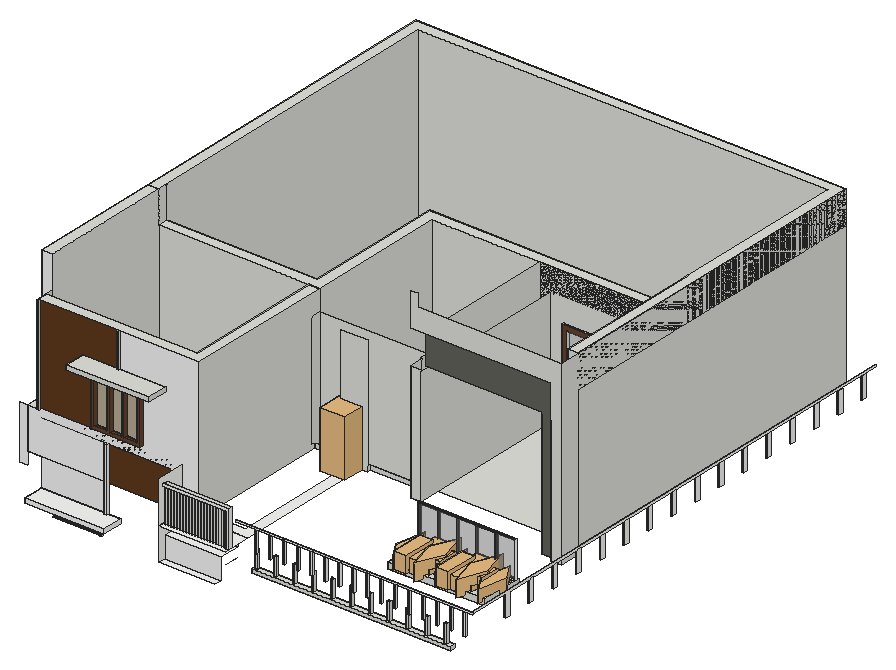
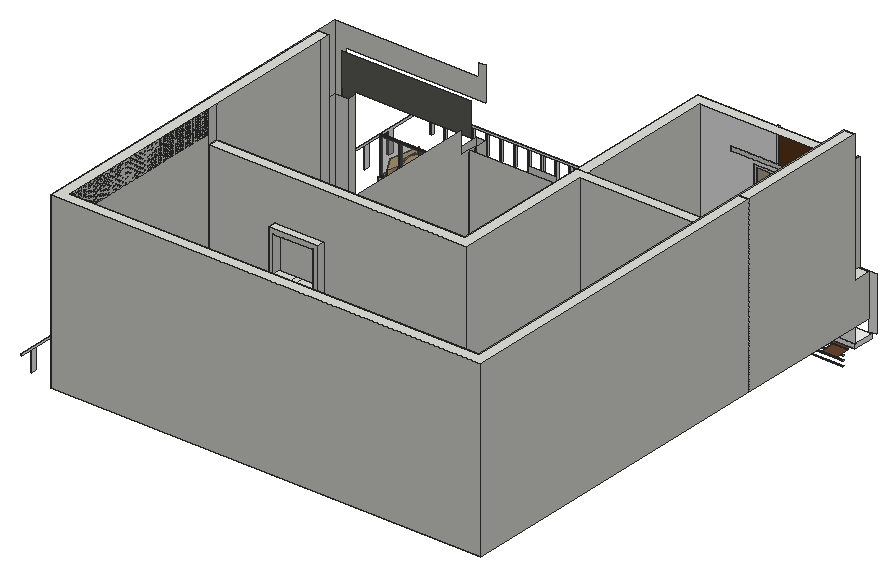
# SketchUp Ruby script. Lengths in inches.
U = 1.inch
M = Sketchup.active_model
def pt(a) = Geom::Point3d.new(a.map { |v| v * U })
def face(e, loops, mat)
  f = e.add_face(loops[0].map { |a| pt(a) })
  loops[1..].each { |l| e.add_face(l.map { |a| pt(a) }).erase! }
  f.material = f.back_material = mat if mat
  f
end
# faces: each face lists its corners as indices into pts; further lists are holes
def faces(e, pts, list, mat = nil) = list.each { |f| face(e, (f[0].is_a?(Array) ? f : [f]).map { |l| l.map { |i| pts[i] } }, mat) }
# xy, xz, yz: faces in a plane at the given z, y or x. An outline is a flat list of corners, or four numbers for a rectangle; further outlines are holes
def ring(l) = l.size == 4 ? [[l[0], l[1]], [l[2], l[1]], [l[2], l[3]], [l[0], l[3]]] : l.each_slice(2).to_a
def flat(e, list, mat, &to3) = list.each { |f| face(e, (f[0].is_a?(Array) ? f : [f]).map { |l| ring(l).map { |u, v| to3.(u, v) } }, mat) }
def xy(e, z, list, mat = nil) = flat(e, list, mat) { |x, y| [x, y, z] }
def xz(e, y, list, mat = nil) = flat(e, list, mat) { |x, z| [x, y, z] }
def yz(e, x, list, mat = nil) = flat(e, list, mat) { |y, z| [x, y, z] }
def lines(e, pts, list) = list.each { |a, b| e.add_line(pt(pts[a]), pt(pts[b])) }
# prism: a flat outline (further loops are holes) pulled along v
def prism(e, loops, v, mat = nil)
  f = face(e, loops, mat); d = Geom::Vector3d.new(v.map { |x| x * U })
  f.pushpull(f.normal.samedirection?(d) ? d.length : -d.length)
end
def box(e, o, s, mat = nil) = prism(e, [[o, [o[0] + s[0], o[1], o[2]], [o[0] + s[0], o[1] + s[1], o[2]], [o[0], o[1] + s[1], o[2]]]], [0, 0, s[2]], mat)
def at(x, y, z, deg = 0) = Geom::Transformation.translation(pt([x, y, z])) * Geom::Transformation.rotation(ORIGIN, Z_AXIS, deg.degrees)
def axes(o, x, y, z) = Geom::Transformation.new([*x, 0, *y, 0, *z, 0, *pt(o).to_a, 1])
def part(name) = M.definitions.add(name)
# library, detail: a bought-in or finely detailed component or shape, given as its bounding box
def library(name, o, s) = part(name).tap { |d| box(d.entities, o, s) }
def detail(e, o, s) = box(e.add_group.entities, o, s)
def put(e, d, t, mat = nil) = e.add_instance(d, t).tap { |i| i.material = mat if mat }
def group(e, t, mat = nil) = e.add_group.tap { |g| g.transformation = t; g.material = mat if mat }.entities
root = M.entities
M.materials.add("ARMANI GRIS").color = [109, 100, 95]
M.materials.add("Brick_21_1K").color = [96, 58, 28]
M.materials.add("CALACATA").color = [248, 248, 247]
M.materials.add("Glass_Basic_01").color = [161, 173, 186]
M.materials["Glass_Basic_01"].alpha = 0.25
M.materials.add("Glass_Mirror_1").color = [185, 173, 151]
M.materials.add("Glass_Safety_01").color = [204, 235, 244]
M.materials["Glass_Safety_01"].alpha = 0.25
M.materials.add("Material__1").color = [95, 70, 46]
M.materials.add("Metal_06_1K").color = [238, 236, 231]
M.materials.add("PIETRA GRAY").color = [98, 99, 92]
M.materials.add("Wood_Veneer_15_1K").color = [103, 69, 45]
M.materials.add("[Color M00]").color = [255, 255, 255]
M.materials.add("[Translucent Glass Gray]").color = [128, 128, 128]
M.materials["[Translucent Glass Gray]"].alpha = 0.29
c1 = library("Group_2",[-1.28,-0.39,0],[21.22,20.51,48.44])
c2 = library("Areca palm plant",[0,0,0],[49.1,36.6,54.46])
c3 = part("W1")
xy(c3.entities,15,[[0,0,2,198]])
xy(c3.entities,102.0625,[[0,0,2,198]],"[Color M00]")
xz(c3.entities,0,[[0,15,2,102.0625]],"[Color M00]")
xz(c3.entities,198,[[0,15,2,102.0625]])
yz(c3.entities,0,[[0.84,16,39.43,101.0625],[40.28,16,78.87,101.0625],[79.71,16,118.3,101.0625],[119.14,16,157.73,101.0625],[158.58,16,197.16,101.0625]])
yz(c3.entities,0,[[[0,15,198,102.0625],[0.84,16,197.16,101.0625]],[39.43,16,40.28,101.0625],[78.87,16,79.71,101.0625],[118.3,16,119.14,101.0625],[157.73,16,158.58,101.0625]],"[Color M00]")
yz(c3.entities,2,[[0.84,16,39.43,101.0625],[40.28,16,78.87,101.0625],[79.71,16,118.3,101.0625],[119.14,16,157.73,101.0625],[158.58,16,197.16,101.0625]])
yz(c3.entities,2,[[[0,15,198,102.0625],[0.84,16,197.16,101.0625]],[39.43,16,40.28,101.0625],[78.87,16,79.71,101.0625],[118.3,16,119.14,101.0625],[157.73,16,158.58,101.0625]],"[Color M00]")
c4 = library("Group\#74",[-84.69,-90.07,-0.36],[176.51,175.13,171.4])
c5 = library("Group20\#1",[-20.81,-17.08,3.79],[39.86,39.43,37.51])
c6 = library("Group\#130",[-7.34,-1.2,0],[38.67,35.81,49.04])
c7 = library("Group38\#2",[14.01,28.44,-23.43],[18.58,18.32,38.89])
c8 = part("PLANTS (1)")
put(c8.entities,c2,axes([38.49,169.84,6.02],[0.45017,-0.56191,0],[0.66137,0.52986,0],[0,0,0.72]))
put(c8.entities,c2,axes([38.49,68.02,6.02],[0.45017,-0.56191,0],[0.66137,0.52986,0],[0,0,0.72]))
put(c8.entities,c3,axes([76.68,11.43,-0.0625],[1,0,0],[0,1.18586,0],[0,0,1]),"[Translucent Glass Gray]")
put(c8.entities,c4,axes([59.61,184.54,5.99],[-0.04961,-0.08593,0],[0.08593,-0.04961,0],[0,0,0.10522]))
put(c8.entities,c4,axes([59.61,204.61,5.99],[-0.04961,-0.08593,0],[0.08593,-0.04961,0],[0,0,0.10522]))
put(c8.entities,c4,axes([59.61,157.29,5.99],[-0.04961,-0.08593,0],[0.08593,-0.04961,0],[0,0,0.10522]))
put(c8.entities,c5,axes([63.65,91.4,4.71],[0,0.85,0],[-0.85,0,0],[0,0,0.85]))
put(c8.entities,c6,axes([69.62,101.34,7.93],[0,0.79,0],[-0.79,0,0],[0,0,0.79]))
put(c8.entities,c7,axes([40.58,10.27,28.11],[0.8848,0,0],[0,0.94674,0],[0,0,0.85826]))
put(c8.entities,c4,axes([59.61,55.48,5.99],[-0.04961,-0.08593,0],[0.08593,-0.04961,0],[0,0,0.10522]))
put(c8.entities,c4,axes([59.61,82.73,5.99],[-0.04961,-0.08593,0],[0.08593,-0.04961,0],[0,0,0.10522]))
put(c8.entities,c4,axes([61.875,132.66,6.01],[-0.08133,-0.14087,0],[0.14087,-0.08133,0],[0,0,0.1725]))
put(c8.entities,c4,axes([59.61,102.79,5.99],[-0.04961,-0.08593,0],[0.08593,-0.04961,0],[0,0,0.10522]))
put(c8.entities,c4,axes([61.875,27.22,6.01],[-0.08133,-0.14087,0],[0.14087,-0.08133,0],[0,0,0.1725]))
put(c8.entities,c4,axes([61.875,234.47,6.01],[-0.08133,-0.14087,0],[0.14087,-0.08133,0],[0,0,0.1725]))
put(c8.entities,c6,axes([69.62,203.15,7.93],[0,0.79,0],[-0.79,0,0],[0,0,0.79]))
put(c8.entities,c5,axes([63.65,193.21,4.71],[0,0.85,0],[-0.85,0,0],[0,0,0.85]))
put(c8.entities,c7,axes([40.58,112.08,28.11],[0.8848,0,0],[0,0.94674,0],[0,0,0.85826]))
g1 = group(c8.entities,at(44.68,11.43,-0.0625))
xy(g1,0,[[0,0,6,234.8],[30,0,36,234.8]])
xy(g1,3,[[6,0,30,234.8]])
xy(g1,7,[[6,5,30,229.8]],"Material__1")
xy(g1,15,[[[0,0,36,234.8],[6,5,30,229.8]]])
xz(g1,0,[[0,0,6,0,6,3,30,3,30,0,36,0,36,15,0,15]])
xz(g1,5,[[6,7,30,15]])
xz(g1,229.8,[[6,7,30,15]])
xz(g1,234.8,[[0,0,0,15,36,15,36,0,30,0,30,3,6,3,6,0]])
yz(g1,0,[[0,0,234.8,15]])
yz(g1,6,[[0,0,234.8,3],[5,7,229.8,15]])
yz(g1,30,[[0,0,234.8,3],[5,7,229.8,15]])
yz(g1,36,[[0,0,234.8,15]])
prism(root,[[[37.375,192.91,86.39],[37.375,193.58,86.39],[79.24,193.58,86.55],[79.24,192.91,86.55]]],[0,0,0.46])
prism(root,[[[37.375,192.91,90.53],[37.375,193.58,90.53],[79.24,193.58,90.69],[79.24,192.91,90.69]]],[0,0,0.46])
prism(root,[[[37.375,192.91,94.67],[37.375,193.58,94.67],[79.24,193.58,94.83],[79.24,192.91,94.83]]],[0,0,0.46])
xy(root,86.45,[[164.8,191.73,168.1,192.23],[168.6,191.73,171.39,192.23],[171.89,191.73,174.68,192.23],[175.18,191.73,177.98,192.23]],"CALACATA")
xy(root,86.95,[[164.8,191.73,168.1,192.23],[168.6,191.73,171.39,192.23],[171.89,191.73,174.68,192.23],[175.18,191.73,177.98,192.23]],"CALACATA")
xy(root,92.29,[[164.8,191.73,168.1,192.23],[168.6,191.73,171.39,192.23],[171.89,191.73,174.68,192.23],[175.18,191.73,177.98,192.23]],"CALACATA")
xy(root,92.79,[[164.8,191.73,168.1,192.23],[168.6,191.73,171.39,192.23],[171.89,191.73,174.68,192.23],[175.18,191.73,177.98,192.23]],"CALACATA")
xy(root,93.95,[[164.8,191.73,168.1,192.23],[168.6,191.73,171.39,192.23],[171.89,191.73,174.68,192.23],[175.18,191.73,177.98,192.23]],"CALACATA")
xy(root,94.45,[[164.8,188.73,177.98,191.73]],"CALACATA")
xy(root,97.45,[[161.8,188.73,180.98,191.73]],"CALACATA")
xy(root,101.97,[[[205.35,195.3125,205.35,199.79,371.5625,199.79,371.875,198.76,369.52,198.76,369.52,196.14,372.66,196.14,371.875,198.76,371.5625,199.79,375.75,199.79,375.75,195.3125],[333.14,196.14,336.28,198.76],[342.23,196.14,345.37,198.76],[351.33,196.14,354.47,198.76],[360.42,196.14,363.5625,198.76]],[342.23,196.14,345.37,198.76],[351.33,196.14,354.47,198.76],[360.42,196.14,363.5625,198.76],[369.52,196.14,369.52,198.76,371.875,198.76,372.66,196.14],
  [369.52,196.14,372.66,198.76]])
xy(root,102,[[148.35,167.73,196.35,173.73]],"CALACATA")
xy(root,102.58,[[28.35,173.73,28.35,191.73,83.14,191.73,83.14,189.73,86.14,189.73,86.14,191.73,96.36,191.73,96.36,173.73],[83.14,189.73,86.14,191.73]],"CALACATA")
xy(root,104.99,[[[205.35,195.3125,375.75,199.79],[320.46,196.77,322.78,198.72],[336.69,196.77,339,198.72],[206.92,196.77,209.24,198.72],[223.14,196.77,225.46,198.72],[239.36,196.77,241.68,198.72],[255.58,196.77,257.9,198.72],[271.8,196.77,274.12,198.72],[288.02,196.77,290.34,198.72],[304.24,196.77,306.5625,198.72],[352.91,196.77,355.22,198.72],[369.125,196.77,371.45,198.72]],[223.14,196.77,225.46,198.72],[239.36,196.77,241.68,198.72],[255.58,196.77,257.9,198.72],[271.8,196.77,274.12,198.72],
  [288.02,196.77,290.34,198.72],[304.24,196.77,306.5625,198.72],[320.46,196.77,322.78,198.72],[336.69,196.77,339,198.72],[352.91,196.77,355.22,198.72],
  [369.125,196.77,371.45,198.72]])
xy(root,106.3,[[28.35,173.73,96.36,173.73,96.36,191.73,86.14,191.73,86.14,189.73,83.14,189.73,83.14,191.73,28.35,191.73],[83.14,189.73,86.14,191.73]],"CALACATA")
xy(root,120,[[206.92,196.77,209.24,198.72],[223.14,196.77,225.46,198.72],[239.36,196.77,241.68,198.72],[255.58,196.77,257.9,198.72],[271.8,196.77,274.12,198.72],
  [288.02,196.77,290.34,198.72],[304.24,196.77,306.5625,198.72],[320.46,196.77,322.78,198.72],[336.69,196.77,339,198.72],[352.91,196.77,355.22,198.72],
  [369.125,196.77,371.45,198.72]])
xy(root,120,[[148.35,173.73,196.35,191.73]],"CALACATA")
xy(root,123.25,[[375.75,302.73,384.75,320.73],[364.23,307.15,375.75,314.04]])
xy(root,130,[[255.75,302.73,264.75,440.73],[188.75,312.0625,188.75,315.0625,163.52,315.0625,163.52,320.73,255.75,320.73,255.75,315.0625,211.23,315.0625,211.23,312.0625]])
xy(root,130,[[[148.35,167.73,205.35,167.73,205.35,171.04,202.67,171.04,202.67,174.71,205.35,174.71,205.35,191.73,148.35,191.73],[150.1875,171.76,151,173.13]],[16.35,191.73,205.35,191.73,205.35,320.73,196.35,320.73,196.35,200.73,25.35,200.73,25.35,320.73,16.35,320.73]],"CALACATA")
xz(root,171.04,[[202.67,130,205.35,130,205.35,161.46,148.35,161.46,148.35,158.66,202.67,158.66]],"CALACATA")
xz(root,171.76,[[150.1875,130,151,158.66],[152.72,130,153.54,158.66],[155.26,130,156.08,158.66],[157.8,130,158.61,158.66],[160.34,130,161.15,158.66],
  [162.875,130,163.6875,158.66],[165.41,130,166.23,158.66],[167.95,130,168.76,158.66],[170.49,130,171.3,158.66],[173.02,130,173.84,158.66],
  [175.56,130,176.375,158.66],[178.1,130,178.91,158.66],[180.63,130,181.45,158.66],[183.17,130,183.99,158.66],[185.71,130,186.52,158.66],
  [188.25,130,189.06,158.66],[190.78,130,191.6,158.66],[193.32,130,194.13,158.66],[195.86,130,196.67,158.66],[198.4,130,199.21,158.66],
  [200.93,130,201.75,158.66]],"CALACATA")
xz(root,173.13,[[150.1875,130,151,158.66],[152.72,130,153.54,158.66],[155.26,130,156.08,158.66],[157.8,130,158.61,158.66],[160.34,130,161.15,158.66],
  [162.875,130,163.6875,158.66],[165.41,130,166.23,158.66],[167.95,130,168.76,158.66],[170.49,130,171.3,158.66],[173.02,130,173.84,158.66],
  [175.56,130,176.375,158.66],[178.1,130,178.91,158.66],[180.63,130,181.45,158.66],[183.17,130,183.99,158.66],[185.71,130,186.52,158.66],
  [188.25,130,189.06,158.66],[190.78,130,191.6,158.66],[193.32,130,194.13,158.66],[195.86,130,196.67,158.66],[198.4,130,199.21,158.66],
  [200.93,130,201.75,158.66]],"CALACATA")
xz(root,173.73,[[148.35,102,196.35,120],[28.35,102.58,96.36,106.3]],"CALACATA")
xz(root,174.71,[[202.67,130,202.67,158.66,148.35,158.66,148.35,161.46,205.35,161.46,205.35,130]],"CALACATA")
xz(root,177.27,[[401.08,130,402.875,148.29]],"CALACATA")
xz(root,177.33,[[389.13,130,390.92,148.29]],"CALACATA")
xz(root,177.39,[[377.17,130,378.97,148.29]],"CALACATA")
xz(root,177.44,[[365.22,130,367.01,148.29]],"CALACATA")
xz(root,177.5,[[353.27,130,355.06,148.29]],"CALACATA")
xz(root,177.56,[[341.3125,130,343.11,148.29]],"CALACATA")
xz(root,177.62,[[329.36,130,331.15,148.29]],"CALACATA")
xz(root,177.68,[[317.41,130,319.2,148.29]],"CALACATA")
xz(root,177.73,[[305.45,130,307.25,148.29]],"CALACATA")
xz(root,177.79,[[293.5,130,295.29,148.29]],"CALACATA")
xz(root,177.85,[[281.55,130,283.34,148.29]],"CALACATA")
xz(root,177.91,[[269.59,130,271.39,148.29]],"CALACATA")
xz(root,177.96,[[257.64,130,259.43,148.29]],"CALACATA")
xz(root,178.02,[[245.6875,130,247.48,148.29]],"CALACATA")
xz(root,178.08,[[233.73,130,235.53,148.29]],"CALACATA")
xz(root,178.14,[[221.78,130,223.57,130,223.57,148.29,408.52,148.29,408.52,149.57,205.35,149.57,205.35,148.29,221.78,148.29]],"CALACATA")
xz(root,178.65,[[401.08,130,402.875,148.29]],"CALACATA")
xz(root,178.7,[[389.13,130,390.92,148.29]],"CALACATA")
xz(root,178.76,[[377.17,130,378.97,148.29]],"CALACATA")
xz(root,178.82,[[365.22,130,367.01,148.29]],"CALACATA")
xz(root,178.875,[[353.27,130,355.06,148.29]],"CALACATA")
xz(root,178.93,[[341.3125,130,343.11,148.29]],"CALACATA")
xz(root,178.99,[[329.36,130,331.15,148.29]],"CALACATA")
xz(root,179.05,[[317.41,130,319.2,148.29]],"CALACATA")
xz(root,179.11,[[305.45,130,307.25,148.29]],"CALACATA")
xz(root,179.17,[[293.5,130,295.29,148.29]],"CALACATA")
xz(root,179.22,[[281.55,130,283.34,148.29]],"CALACATA")
xz(root,179.28,[[269.59,130,271.39,148.29]],"CALACATA")
xz(root,179.34,[[257.64,130,259.43,148.29]],"CALACATA")
xz(root,179.4,[[245.6875,130,247.48,148.29]],"CALACATA")
xz(root,179.46,[[233.73,130,235.53,148.29]],"CALACATA")
xz(root,179.51,[[221.78,130,221.78,148.29,205.35,148.29,205.35,149.57,406.51,149.57,406.51,148.29,223.57,148.29,223.57,130]],"CALACATA")
xz(root,189.73,[[83.14,106.3,86.14,160]],"CALACATA")
xz(root,191.73,[[171.39,86.45,171.89,86.95],[174.68,86.45,175.18,86.95],[28.35,102.58,83.14,106.3],[83.14,102.58,86.14,106.3,83.14,106.3],[83.14,102.58,96.36,102.58,96.36,106.3,86.14,106.3],
  [28.35,106.3,83.14,130],[83.14,106.3,86.14,130],[10.35,120,10.35,166,139.35,166,139.35,160,28.35,160,28.35,130,16.35,130,16.35,120],[148.35,120,196.35,130],[83.14,130,86.14,160],
  [139.35,130,148.35,166]],"CALACATA")
xz(root,191.73,[[164.8,86.45,168.1,86.95],[168.1,86.45,168.6,86.95],[168.6,86.45,171.39,86.95],[171.89,86.45,174.68,86.95],[175.18,86.45,177.98,86.95],
  [168.1,86.95,168.6,92.29],[171.39,86.95,171.89,92.29],[174.68,86.95,175.18,92.29],[164.8,92.29,168.1,92.79],[168.1,92.29,168.6,92.79],
  [168.6,92.29,171.39,92.79],[171.39,92.29,171.89,92.79],[171.89,92.29,174.68,92.79],[174.68,92.29,175.18,92.79],[175.18,92.29,177.98,92.79],
  [168.1,92.79,168.6,93.95],[171.39,92.79,171.89,93.95],[174.68,92.79,175.18,93.95],[164.8,93.95,168.1,94.45],[168.1,93.95,168.6,94.45],
  [168.6,93.95,171.39,94.45],[171.39,93.95,171.89,94.45],[171.89,93.95,174.68,94.45],[174.68,93.95,175.18,94.45],[175.18,93.95,177.98,94.45]],"Metal_06_1K")
xz(root,192.23,[[164.8,86.95,168.1,92.29],[168.6,86.95,171.39,92.29],[171.89,86.95,174.68,92.29],[175.18,86.95,177.98,92.29],[164.8,92.79,168.1,93.95],
  [168.6,92.79,171.39,93.95],[171.89,92.79,174.68,93.95],[175.18,92.79,177.98,93.95]],"Glass_Safety_01")
xz(root,195.3125,[[205.35,101.97,375.75,104.99]])
xz(root,196.77,[[206.92,104.99,209.24,120],[223.14,104.99,225.46,120],[239.36,104.99,241.68,120],[255.58,104.99,257.9,120],[271.8,104.99,274.12,120],
  [288.02,104.99,290.34,120],[304.24,104.99,306.5625,120],[320.46,104.99,322.78,120],[336.69,104.99,339,120],[352.91,104.99,355.22,120],
  [369.125,104.99,371.45,120]])
xz(root,198.72,[[206.92,104.99,209.24,120],[223.14,104.99,225.46,120],[239.36,104.99,241.68,120],[255.58,104.99,257.9,120],[271.8,104.99,274.12,120],
  [288.02,104.99,290.34,120],[304.24,104.99,306.5625,120],[320.46,104.99,322.78,120],[336.69,104.99,339,120],[352.91,104.99,355.22,120],
  [369.125,104.99,371.45,120]])
xz(root,199.79,[[205.35,101.97,375.75,104.99]])
xz(root,214.38,[[406.51,130,407.89,148.29]],"CALACATA")
xz(root,218.18,[[406.51,130,407.89,148.29]],"CALACATA")
xz(root,239.75,[[406.57,130,407.94,148.29]],"CALACATA")
xz(root,243.56,[[406.57,130,407.94,148.29]],"CALACATA")
xz(root,265.12,[[406.625,130,408,148.29]],"CALACATA")
xz(root,268.93,[[406.625,130,408,148.29]],"CALACATA")
xz(root,290.49,[[406.68,130,408.06,148.29]],"CALACATA")
xz(root,294.3,[[406.68,130,408.06,148.29]],"CALACATA")
xz(root,302.73,[[375.75,123.25,384.75,123.25,384.75,278,261.75,278,261.75,288.73,255.75,288.73,255.75,260,375.75,260],[255.75,130,264.75,231.11]])
xz(root,307.15,[[364.23,123.25,375.75,123.25,375.75,260,264.75,260,264.75,232,364.23,232]],"PIETRA GRAY")
xz(root,312.0625,[[188.75,130,211.23,231.11]])
xz(root,314.04,[[364.23,123.25,375.75,229.58]])
xz(root,315.0625,[[163.52,130,188.75,134.25],[211.23,130,255.75,130,255.75,231.11,254.75,231.11,254.75,134.12,211.23,134.12]])
xz(root,315.86,[[406.74,130,408.12,148.29]],"CALACATA")
xz(root,319.67,[[406.74,130,408.12,148.29]],"CALACATA")
xz(root,320.73,[[375.75,123.25,384.75,250],[163.52,130,255.75,232]])
xz(root,341.23,[[406.8,130,408.17,148.29]],"CALACATA")
xz(root,345.04,[[406.8,130,408.17,148.29]],"CALACATA")
xz(root,366.61,[[406.86,130,408.23,148.29]],"CALACATA")
xz(root,370.41,[[406.86,130,408.23,148.29]],"CALACATA")
xz(root,391.98,[[406.92,130,408.29,148.29]],"CALACATA")
xz(root,395.78,[[406.92,130,408.29,148.29]],"CALACATA")
xz(root,417.35,[[406.97,130,408.35,148.29]],"CALACATA")
xz(root,421.15,[[406.97,130,408.35,148.29]],"CALACATA")
xz(root,440.73,[[255.75,130,255.75,250,375.75,250,375.75,229.58,362.5,229.58,362.5,231.11,268.75,231.11,268.75,229.63,264.75,229.63,264.75,130]])
xz(root,442.72,[[407.03,130,408.41,148.29]],"CALACATA")
xz(root,446.52,[[407.03,130,408.41,148.29]],"CALACATA")
xz(root,468.09,[[407.09,130,408.46,148.29]],"CALACATA")
xz(root,471.89,[[407.09,130,408.46,148.29]],"CALACATA")
xz(root,493.46,[[407.15,130,408.52,148.29]],"CALACATA")
xz(root,497.27,[[407.15,130,408.52,148.29]],"CALACATA")
xz(root,518.83,[[407.2,130,408.58,148.29]],"CALACATA")
xz(root,522.64,[[407.2,130,408.58,148.29]],"CALACATA")
xz(root,544.2,[[407.26,130,408.64,148.29]],"CALACATA")
xz(root,548.01,[[407.26,130,408.64,148.29]],"CALACATA")
xz(root,569.57,[[407.32,130,408.69,148.29]],"CALACATA")
xz(root,573.38,[[407.32,130,408.69,148.29]],"CALACATA")
xz(root,594.94,[[407.38,130,408.75,148.29]],"CALACATA")
xz(root,598.75,[[407.38,130,408.75,148.29]],"CALACATA")
yz(root,28.35,[[173.73,102.58,191.73,105.96],[173.73,105.96,191.73,106.3]],"CALACATA")
yz(root,49.82,[[188.73,97.34,200.73,97.4]],"CALACATA")
yz(root,52.82,[[188.73,97.35,200.73,97.41]],"CALACATA")
yz(root,63.77,[[188.73,97.36,200.73,97.45]],"CALACATA")
yz(root,66.77,[[188.73,97.36,200.73,97.47]],"CALACATA")
yz(root,79.23,[[188.73,97.35,200.73,97.51]],"CALACATA")
yz(root,83.14,[[189.73,106.3,191.73,160]],"CALACATA")
yz(root,86.14,[[189.73,106.3,191.73,160]],"CALACATA")
yz(root,96.36,[[173.73,102.58,191.73,106.3]],"CALACATA")
yz(root,148.35,[[167.73,102,167.73,130,191.73,130,191.73,120,173.73,120,173.73,102],[[167.73,130,191.73,166],[171.04,158.66,174.71,161.46]]],"CALACATA")
yz(root,150.1875,[[171.76,130,173.13,158.66]],"CALACATA")
yz(root,151,[[171.76,130,173.13,158.66]],"CALACATA")
yz(root,152.72,[[171.76,130,173.13,158.66]],"CALACATA")
yz(root,153.54,[[171.76,130,173.13,158.66]],"CALACATA")
yz(root,155.26,[[171.76,130,173.13,158.66]],"CALACATA")
yz(root,156.08,[[171.76,130,173.13,158.66]],"CALACATA")
yz(root,157.8,[[171.76,130,173.13,158.66]],"CALACATA")
yz(root,158.61,[[171.76,130,173.13,158.66]],"CALACATA")
yz(root,160.34,[[171.76,130,173.13,158.66]],"CALACATA")
yz(root,161.15,[[171.76,130,173.13,158.66]],"CALACATA")
yz(root,162.875,[[171.76,130,173.13,158.66]],"CALACATA")
yz(root,163.52,[[315.0625,130,315.0625,134.25,312.0625,134.25,312.0625,232,320.73,232,320.73,130]])
yz(root,163.6875,[[171.76,130,173.13,158.66]],"CALACATA")
yz(root,165.41,[[171.76,130,173.13,158.66]],"CALACATA")
yz(root,166.23,[[171.76,130,173.13,158.66]],"CALACATA")
yz(root,167.95,[[171.76,130,173.13,158.66]],"CALACATA")
yz(root,168.1,[[191.73,86.95,192.23,92.29],[191.73,92.79,192.23,93.95]],"CALACATA")
yz(root,168.6,[[191.73,86.95,192.23,92.29],[191.73,92.79,192.23,93.95]],"CALACATA")
yz(root,168.76,[[171.76,130,173.13,158.66]],"CALACATA")
yz(root,170.49,[[171.76,130,173.13,158.66]],"CALACATA")
yz(root,171.3,[[171.76,130,173.13,158.66]],"CALACATA")
yz(root,171.39,[[191.73,86.95,192.23,92.29],[191.73,92.79,192.23,93.95]],"CALACATA")
yz(root,171.89,[[191.73,86.95,192.23,92.29],[191.73,92.79,192.23,93.95]],"CALACATA")
yz(root,173.02,[[171.76,130,173.13,158.66]],"CALACATA")
yz(root,173.84,[[171.76,130,173.13,158.66]],"CALACATA")
yz(root,174.68,[[191.73,86.95,192.23,92.29],[191.73,92.79,192.23,93.95]],"CALACATA")
yz(root,175.18,[[191.73,86.95,192.23,92.29],[191.73,92.79,192.23,93.95]],"CALACATA")
yz(root,175.56,[[171.76,130,173.13,158.66]],"CALACATA")
yz(root,176.375,[[171.76,130,173.13,158.66]],"CALACATA")
yz(root,178.1,[[171.76,130,173.13,158.66]],"CALACATA")
yz(root,178.91,[[171.76,130,173.13,158.66]],"CALACATA")
yz(root,180.63,[[171.76,130,173.13,158.66]],"CALACATA")
yz(root,181.45,[[171.76,130,173.13,158.66]],"CALACATA")
yz(root,183.17,[[171.76,130,173.13,158.66]],"CALACATA")
yz(root,183.99,[[171.76,130,173.13,158.66]],"CALACATA")
yz(root,185.71,[[171.76,130,173.13,158.66]],"CALACATA")
yz(root,186.52,[[171.76,130,173.13,158.66]],"CALACATA")
yz(root,188.25,[[171.76,130,173.13,158.66]],"CALACATA")
yz(root,188.75,[[312.0625,130,315.0625,134.25]])
yz(root,189.06,[[171.76,130,173.13,158.66]],"CALACATA")
yz(root,190.78,[[171.76,130,173.13,158.66]],"CALACATA")
yz(root,191.6,[[171.76,130,173.13,158.66]],"CALACATA")
yz(root,193.32,[[171.76,130,173.13,158.66]],"CALACATA")
yz(root,194.13,[[171.76,130,173.13,158.66]],"CALACATA")
yz(root,195.86,[[171.76,130,173.13,158.66]],"CALACATA")
yz(root,196.67,[[171.76,130,173.13,158.66]],"CALACATA")
yz(root,198.4,[[171.76,130,173.13,158.66]],"CALACATA")
yz(root,199.21,[[171.76,130,173.13,158.66]],"CALACATA")
yz(root,200.93,[[171.76,130,173.13,158.66]],"CALACATA")
yz(root,201.75,[[171.76,130,173.13,158.66]],"CALACATA")
yz(root,202.67,[[171.04,130,174.71,158.66]],"CALACATA")
yz(root,205.35,[[195.3125,101.97,199.79,104.99]])
yz(root,205.35,[[171.04,130,174.71,161.46]],"CALACATA")
yz(root,206.92,[[196.77,104.99,198.72,120]])
yz(root,209.24,[[196.77,104.99,198.72,120]])
yz(root,211.23,[[312.0625,130,315.0625,134.12]])
yz(root,221.78,[[178.14,130,179.51,148.29]],"CALACATA")
yz(root,223.14,[[196.77,104.99,198.72,120]])
yz(root,223.57,[[178.14,130,179.51,148.29]],"CALACATA")
yz(root,225.46,[[196.77,104.99,198.72,120]])
yz(root,233.73,[[178.08,130,179.46,148.29]],"CALACATA")
yz(root,235.53,[[178.08,130,179.46,148.29]],"CALACATA")
yz(root,239.36,[[196.77,104.99,198.72,120]])
yz(root,241.68,[[196.77,104.99,198.72,120]])
yz(root,245.6875,[[178.02,130,179.4,148.29]],"CALACATA")
yz(root,247.48,[[178.02,130,179.4,148.29]],"CALACATA")
yz(root,255.58,[[196.77,104.99,198.72,120]])
yz(root,255.75,[[302.73,130,315.0625,231.11],[315.0625,130,320.73,232],[320.73,130,320.73,232,329.73,232,329.73,250,440.73,250,440.73,130]])
yz(root,257.64,[[177.96,130,179.34,148.29]],"CALACATA")
yz(root,257.9,[[196.77,104.99,198.72,120]])
yz(root,259.43,[[177.96,130,179.34,148.29]],"CALACATA")
yz(root,264.75,[[302.73,130,440.73,229.63]])
yz(root,269.59,[[177.91,130,179.28,148.29]],"CALACATA")
yz(root,271.39,[[177.91,130,179.28,148.29]],"CALACATA")
yz(root,271.8,[[196.77,104.99,198.72,120]])
yz(root,274.12,[[196.77,104.99,198.72,120]])
yz(root,281.55,[[177.85,130,179.22,148.29]],"CALACATA")
yz(root,283.34,[[177.85,130,179.22,148.29]],"CALACATA")
yz(root,288.02,[[196.77,104.99,198.72,120]])
yz(root,290.34,[[196.77,104.99,198.72,120]])
yz(root,293.5,[[177.79,130,179.17,148.29]],"CALACATA")
yz(root,295.29,[[177.79,130,179.17,148.29]],"CALACATA")
yz(root,304.24,[[196.77,104.99,198.72,120]])
yz(root,305.45,[[177.73,130,179.11,148.29]],"CALACATA")
yz(root,306.5625,[[196.77,104.99,198.72,120]])
yz(root,307.25,[[177.73,130,179.11,148.29]],"CALACATA")
yz(root,317.41,[[177.68,130,179.05,148.29]],"CALACATA")
yz(root,319.2,[[177.68,130,179.05,148.29]],"CALACATA")
yz(root,320.46,[[196.77,104.99,198.72,120]])
yz(root,322.78,[[196.77,104.99,198.72,120]])
yz(root,329.36,[[177.62,130,178.99,148.29]],"CALACATA")
yz(root,331.15,[[177.62,130,178.99,148.29]],"CALACATA")
yz(root,336.69,[[196.77,104.99,198.72,120]])
yz(root,339,[[196.77,104.99,198.72,120]])
yz(root,341.3125,[[177.56,130,178.93,148.29]],"CALACATA")
yz(root,343.11,[[177.56,130,178.93,148.29]],"CALACATA")
yz(root,352.91,[[196.77,104.99,198.72,120]])
yz(root,353.27,[[177.5,130,178.875,148.29]],"CALACATA")
yz(root,355.06,[[177.5,130,178.875,148.29]],"CALACATA")
yz(root,355.22,[[196.77,104.99,198.72,120]])
yz(root,364.23,[[307.15,123.25,314.04,229.58]])
yz(root,365.22,[[177.44,130,178.82,148.29]],"CALACATA")
yz(root,367.01,[[177.44,130,178.82,148.29]],"CALACATA")
yz(root,369.125,[[196.77,104.99,198.72,120]])
yz(root,371.45,[[196.77,104.99,198.72,120]])
yz(root,375.75,[[195.3125,101.97,199.79,104.99],[302.73,123.25,307.15,231.11],[314.04,123.25,320.73,229.58]])
yz(root,377.17,[[177.39,130,178.76,148.29]],"CALACATA")
yz(root,378.97,[[177.39,130,178.76,148.29]],"CALACATA")
yz(root,384.75,[[302.73,123.25,320.73,123.25,320.73,250,607.49,250,607.49,278,302.73,278]])
yz(root,389.13,[[177.33,130,178.7,148.29]],"CALACATA")
yz(root,390.92,[[177.33,130,178.7,148.29]],"CALACATA")
yz(root,401.08,[[177.27,130,178.65,148.29]],"CALACATA")
yz(root,402.875,[[177.27,130,178.65,148.29]],"CALACATA")
yz(root,406.51,[[214.38,130,214.38,148.29,179.51,148.29,179.51,149.57,610.73,149.57,610.73,148.29,218.18,148.29,218.18,130]],"CALACATA")
yz(root,406.57,[[239.75,130,243.56,148.29]],"CALACATA")
yz(root,406.625,[[265.12,130,268.93,148.29]],"CALACATA")
yz(root,406.68,[[290.49,130,294.3,148.29]],"CALACATA")
yz(root,406.74,[[315.86,130,319.67,148.29]],"CALACATA")
yz(root,406.8,[[341.23,130,345.04,148.29]],"CALACATA")
yz(root,406.86,[[366.61,130,370.41,148.29]],"CALACATA")
yz(root,406.92,[[391.98,130,395.78,148.29]],"CALACATA")
yz(root,406.97,[[417.35,130,421.15,148.29]],"CALACATA")
yz(root,407.03,[[442.72,130,446.52,148.29]],"CALACATA")
yz(root,407.09,[[468.09,130,471.89,148.29]],"CALACATA")
yz(root,407.15,[[493.46,130,497.27,148.29]],"CALACATA")
yz(root,407.2,[[518.83,130,522.64,148.29]],"CALACATA")
yz(root,407.26,[[544.2,130,548.01,148.29]],"CALACATA")
yz(root,407.32,[[569.57,130,573.38,148.29]],"CALACATA")
yz(root,407.38,[[594.94,130,598.75,148.29]],"CALACATA")
yz(root,407.89,[[214.38,130,218.18,130,218.18,148.29,610.73,148.29,610.73,149.57,179.51,149.57,179.51,148.29,214.38,148.29]],"CALACATA")
yz(root,407.94,[[239.75,130,243.56,148.29]],"CALACATA")
yz(root,408,[[265.12,130,268.93,148.29]],"CALACATA")
yz(root,408.06,[[290.49,130,294.3,148.29]],"CALACATA")
yz(root,408.12,[[315.86,130,319.67,148.29]],"CALACATA")
yz(root,408.17,[[341.23,130,345.04,148.29]],"CALACATA")
yz(root,408.23,[[366.61,130,370.41,148.29]],"CALACATA")
yz(root,408.29,[[391.98,130,395.78,148.29]],"CALACATA")
yz(root,408.35,[[417.35,130,421.15,148.29]],"CALACATA")
yz(root,408.41,[[442.72,130,446.52,148.29]],"CALACATA")
yz(root,408.46,[[468.09,130,471.89,148.29]],"CALACATA")
yz(root,408.52,[[493.46,130,497.27,148.29]],"CALACATA")
yz(root,408.58,[[518.83,130,522.64,148.29]],"CALACATA")
yz(root,408.64,[[544.2,130,548.01,148.29]],"CALACATA")
yz(root,408.69,[[569.57,130,573.38,148.29]],"CALACATA")
yz(root,408.75,[[594.94,130,598.75,148.29]],"CALACATA")
p = [[37.36,200.73,97.35],[49.82,200.73,97.4],[49.82,188.73,97.4],[37.36,188.73,97.35],[52.82,188.73,97.41],[52.82,200.73,97.41],
  [63.77,200.73,97.45],[63.77,188.73,97.45],[66.77,188.73,97.47],[66.77,200.73,97.47],[79.23,200.73,97.51],[79.23,188.73,97.51],
  [82.22,191.73,100.52],[34.35,191.73,100.34],[34.35,188.73,100.34],[82.22,188.73,100.52],[49.82,188.73,97.4],[52.82,188.73,97.4],
  [49.82,191.73,97.34],[52.82,191.73,97.34],[205.35,167.73,120],[205.35,179.73,120],[264.94,449.73,250],[264.75,440.73,130],
  [82.35,191.73,100.52],[156.53,173.13,130],[156.53,171.76,130],[157.34,171.76,130],[157.34,173.13,130]]
faces(root,p,[[0,1,2,3],[4,5,6,7],[8,9,10,11],[12,13,14,15]],"Wood_Veneer_15_1K")
lines(root,p,[[16,17],[18,19],[20,21],[22,23],[24,12],[25,26],[27,28]])
g2 = group(root,at(206.92,196.77,104.99))
p = [[0,0,0],[0,1.95,0],[2.32,0,0],[2.32,1.95,0]]
lines(g2,p,[[0,1],[2,0],[3,2],[1,3]])
put(root,c1,at(186.66,293.6,130))
g3 = group(root,at(16.35,320.73,130))
xy(g3,0,[[0,0,147.17,0,147.17,120,359.4,120,359.4,0,368.4,0,368.4,286.76,0,286.76],[147.17,0,359.4,120]])
xy(g3,120,[[9,0,147.17,0,147.17,120,359.4,120,359.4,129,137.78,129,137.78,9,9,9]])
xy(g3,148,[[0,0,9,0,9,277.76,359.4,277.76,359.4,0,368.4,0,368.4,286.76,0,286.76]])
xz(g3,0,[[0,0,9,148],[9,0,147.17,120],[359.4,0,368.4,148]])
xz(g3,9,[[9,0,137.78,120]])
xz(g3,120,[[147.17,0,311.4,0,311.4,101.11,346.15,101.11,346.15,99.58,359.4,99.58,359.4,120,147.17,120]])
xz(g3,120,[[311.4,0,359.4,0,359.4,99.58,346.15,99.58,346.15,101.11,311.4,101.11]],"ARMANI GRIS")
xz(g3,129,[[137.78,0,359.4,120]])
xz(g3,277.76,[[9,0,359.4,148]])
xz(g3,286.76,[[0,0,368.4,148]])
yz(g3,0,[[0,0,286.76,148]])
yz(g3,9,[[9,0,277.76,148],[0,120,9,148]])
yz(g3,137.78,[[9,0,129,120]])
yz(g3,147.17,[[0,0,120,120]])
yz(g3,359.4,[[0,0,9,148],[9,0,120,148],[120,0,129,120],[120,120,129,148]])
yz(g3,368.4,[[0,0,286.76,148]])
p = [[359.4,129,0],[359.4,277.76,0]]
lines(g3,p,[[0,1]])
g4 = group(root,at(16.35,191.73,130))
xy(g4,0,[[0,0,147.17,0,147.17,129,138.17,129,138.17,9,9,9,9,129,0,129],[9,9,138.17,129]])
xy(g4,36,[[9,-1,11,0],[0,0,9,15.58]])
xy(g4,39,[[57,-3,99,0]])
xy(g4,41.5,[[59.5,-3,70.53,0],[73.03,-3,82.92,0],[85.42,-3,96.5,0]],"Wood_Veneer_15_1K")
xy(g4,41.65,[[260.3,247,302.37,264.96]])
xy(g4,45.65,[[264.3,247,279.33,249],[279.33,247,283.33,264.96],[283.33,247,298.37,249],[264.3,249,279.33,264.96],[283.33,249,298.37,264.96]])
xy(g4,76.48,[[264.3,247,279.33,249],[279.33,247,283.33,264.96],[283.33,247,298.37,249],[264.3,249,279.33,264.96],[283.33,249,298.37,264.96]])
xy(g4,80.48,[[260.3,247,302.37,264.96]])
xy(g4,81.5,[[59.5,-3,70.53,0],[73.03,-3,82.92,0],[85.42,-3,96.5,0]],"Wood_Veneer_15_1K")
xy(g4,84,[[57,-3,99,0]],"Wood_Veneer_15_1K")
xy(g4,87,[[47.74,-18,118.15,0]])
xy(g4,91,[[47.74,-18,118.15,-18,118.15,0,79.29,0,79.29,-1,77.29,-1,77.29,0,47.74,0],[77.29,-1,79.29,0]])
xy(g4,120,[[9,-1,11,-1,11,0,77.29,0,77.29,-1,79.29,-1,79.29,0,147.17,0,147.17,129,138.17,129,138.17,9,9,9]])
xy(g4,148,[[0,15.58,9,129]])
xz(g4,-18,[[47.74,87,118.15,91]])
xz(g4,-3,[[[57,39,99,84],[85.42,41.5,96.5,81.5],[59.5,41.5,70.53,81.5],[73.03,41.5,82.92,81.5]]],"Wood_Veneer_15_1K")
xz(g4,-1,[[9,36,11,120],[77.29,91,79.29,120]])
xz(g4,0,[[[57,39,99,84],[85.42,41.5,96.5,81.5],[59.5,41.5,70.53,81.5],[73.03,41.5,82.92,81.5]],[47.74,87,118.15,91]])
xz(g4,0,[[69.79,0,123,30],[11,37.03,57,37.03,57,87,47.74,87,47.74,91,77.29,91,77.29,120,11,120]],"Brick_21_1K")
xz(g4,0,[[0,0,69.79,0,69.79,30,123,30,123,0,147.17,0,147.17,120,79.29,120,79.29,91,118.15,91,118.15,87,57,87,57,84,99,84,99,39,57,39,57,37.03,11,37.03,11,36,0,36]],"CALACATA")
xz(g4,0,[[59.5,41.5,70.53,81.5],[73.03,41.5,82.92,81.5],[85.42,41.5,96.5,81.5]],"Glass_Mirror_1")
xz(g4,15.58,[[0,36,9,148]],"CALACATA")
xz(g4,129,[[0,0,9,148],[138.17,0,147.17,120]])
xz(g4,247,[[[260.3,41.65,302.37,80.48],[264.3,45.65,298.37,76.48]],[279.33,45.65,283.33,76.48]],"Wood_Veneer_15_1K")
xz(g4,249,[[264.3,45.65,279.33,76.48],[283.33,45.65,298.37,76.48]],"Glass_Basic_01")
xz(g4,264.96,[[[260.3,41.65,302.37,80.48],[264.3,45.65,298.37,76.48]]])
yz(g4,0,[[0,0,0,36,15.58,36,15.58,148,129,148,129,0]])
yz(g4,9,[[9,0,129,0,129,148,15.58,148,15.58,36,9,36],[-1,36,15.58,120]])
yz(g4,11,[[-1,36,0,120]])
yz(g4,47.74,[[-18,87,0,91]])
yz(g4,57,[[-3,39,0,84]])
yz(g4,59.5,[[-3,41.5,0,81.5]],"Wood_Veneer_15_1K")
yz(g4,70.53,[[-3,41.5,0,81.5]])
yz(g4,73.03,[[-3,41.5,0,81.5]],"Wood_Veneer_15_1K")
yz(g4,77.29,[[-1,91,0,120]])
yz(g4,79.29,[[-1,91,0,120]])
yz(g4,82.92,[[-3,41.5,0,81.5]])
yz(g4,85.42,[[-3,41.5,0,81.5]],"Wood_Veneer_15_1K")
yz(g4,96.5,[[-3,41.5,0,81.5]])
yz(g4,99,[[-3,39,0,84]],"Wood_Veneer_15_1K")
yz(g4,118.15,[[-18,87,0,91]])
yz(g4,138.17,[[9,0,129,120]])
yz(g4,147.17,[[0,0,129,120]])
yz(g4,260.3,[[247,41.65,264.96,80.48]])
yz(g4,264.3,[[247,45.65,249,76.48],[249,45.65,264.96,76.48]])
yz(g4,279.33,[[247,45.65,249,76.48]])
yz(g4,283.33,[[247,45.65,249,76.48]])
yz(g4,298.37,[[247,45.65,249,76.48],[249,45.65,264.96,76.48]])
yz(g4,302.37,[[247,41.65,264.96,80.48]])
p = [[147.17,129,0],[368.4,129,0],[55,0,36],[53,0,36],[57,0,36],[57,0,37.03],
  [12,0,30],[66.79,0,30]]
lines(g4,p,[[0,1],[2,3],[4,5],[6,7]])
put(root,c8,axes([391.21,173.04,130.02],[0,1,0],[-0.352,0,0],[0,0,0.3604]))
